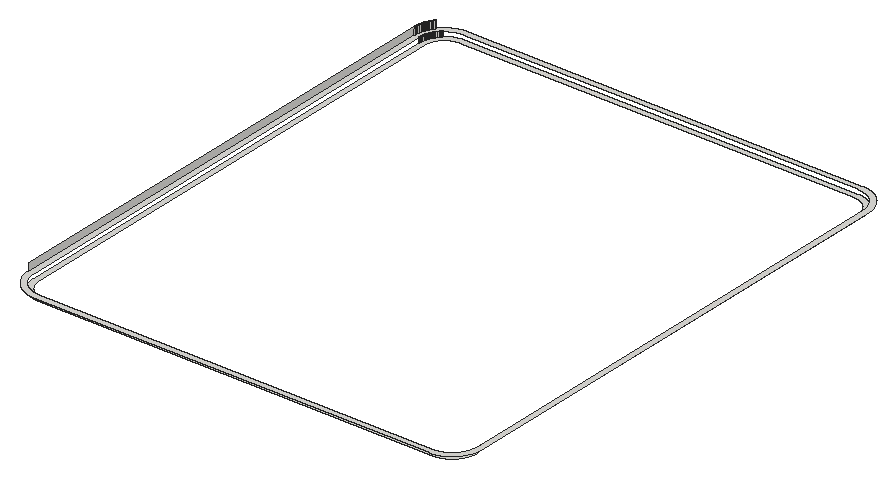
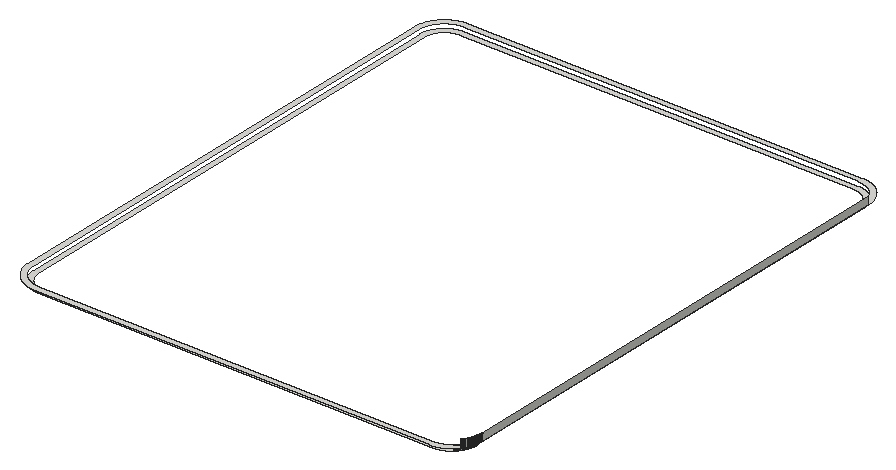
# SketchUp Ruby script. Lengths in inches.
U = 1.inch
M = Sketchup.active_model
def pt(a) = Geom::Point3d.new(a.map { |v| v * U })
def face(e, loops, mat)
  f = e.add_face(loops[0].map { |a| pt(a) })
  loops[1..].each { |l| e.add_face(l.map { |a| pt(a) }).erase! }
  f.material = f.back_material = mat if mat
  f
end
# faces: each face lists its corners as indices into pts; further lists are holes
def faces(e, pts, list, mat = nil) = list.each { |f| face(e, (f[0].is_a?(Array) ? f : [f]).map { |l| l.map { |i| pts[i] } }, mat) }
# xy, xz, yz: faces in a plane at the given z, y or x. An outline is a flat list of corners, or four numbers for a rectangle; further outlines are holes
def ring(l) = l.size == 4 ? [[l[0], l[1]], [l[2], l[1]], [l[2], l[3]], [l[0], l[3]]] : l.each_slice(2).to_a
def flat(e, list, mat, &to3) = list.each { |f| face(e, (f[0].is_a?(Array) ? f : [f]).map { |l| ring(l).map { |u, v| to3.(u, v) } }, mat) }
def xy(e, z, list, mat = nil) = flat(e, list, mat) { |x, y| [x, y, z] }
def xz(e, y, list, mat = nil) = flat(e, list, mat) { |x, z| [x, y, z] }
def yz(e, x, list, mat = nil) = flat(e, list, mat) { |y, z| [x, y, z] }
def lines(e, pts, list) = list.each { |a, b| e.add_line(pt(pts[a]), pt(pts[b])) }
# prism: a flat outline (further loops are holes) pulled along v
def prism(e, loops, v, mat = nil)
  f = face(e, loops, mat); d = Geom::Vector3d.new(v.map { |x| x * U })
  f.pushpull(f.normal.samedirection?(d) ? d.length : -d.length)
end
def box(e, o, s, mat = nil) = prism(e, [[o, [o[0] + s[0], o[1], o[2]], [o[0] + s[0], o[1] + s[1], o[2]], [o[0], o[1] + s[1], o[2]]]], [0, 0, s[2]], mat)
def at(x, y, z, deg = 0) = Geom::Transformation.translation(pt([x, y, z])) * Geom::Transformation.rotation(ORIGIN, Z_AXIS, deg.degrees)
def axes(o, x, y, z) = Geom::Transformation.new([*x, 0, *y, 0, *z, 0, *pt(o).to_a, 1])
def part(name) = M.definitions.add(name)
# library, detail: a bought-in or finely detailed component or shape, given as its bounding box
def library(name, o, s) = part(name).tap { |d| box(d.entities, o, s) }
def detail(e, o, s) = box(e.add_group.entities, o, s)
def put(e, d, t, mat = nil) = e.add_instance(d, t).tap { |i| i.material = mat if mat }
def group(e, t, mat = nil) = e.add_group.tap { |g| g.transformation = t; g.material = mat if mat }.entities
root = M.entities
M.materials.add("[Formica Graystone]").color = [224, 223, 219]
xy(root,422.82,[[[17.74,231,17.61,231.01,17.48,231.01,17.22,231.03,17.08,231.04,16.95,231.05,16.69,231.09,16.57,231.1,16.4375,231.125,16.31,231.14,16.18,231.17,16.05,231.19,15.79,231.25,15.67,231.28,15.41,231.34,15.29,231.375,15.16,231.41,15.03,231.45,14.79,231.53,14.66,231.57,14.54,231.62,14.42,231.66,14.29,231.71,14.17,231.76,14.05,231.8125,13.93,231.86,13.8125,231.92,13.69,231.97,13.58,232.03,13.34,232.15,13.23,232.21,13.11,232.28,13,232.34,12.89,232.41,12.78,232.47,12.66,232.54,12.55,232.61,12.44,232.69,12.34,232.76,12.23,232.83,12.12,232.91,12.02,232.99,11.91,233.07,11.71,233.23,11.61,233.3125,11.51,233.4,11.41,233.48,11.21,233.66,11.12,233.75,11.02,233.84,10.84,234.02,10.75,234.12,10.66,234.21,10.48,234.41,10.4,234.51,10.3125,234.61,10.23,234.71,10.07,234.91,9.99,235.02,9.91,235.12,9.83,235.23,9.76,235.34,9.69,235.44,9.61,235.55,9.54,235.66,9.47,235.78,9.41,235.89,9.34,236,9.28,236.11,9.21,236.23,9.15,236.34,9.03,236.58,8.97,236.69,8.92,236.8125,8.86,236.93,8.8125,237.05,8.76,237.17,8.71,237.29,8.66,237.42,8.62,237.54,8.57,237.66,8.53,237.79,8.45,238.03,8.41,238.16,8.375,238.29,8.34,238.41,8.28,238.67,8.25,238.79,8.19,239.05,8.17,239.18,8.14,239.31,8.125,239.4375,8.1,239.57,8.09,239.69,8.05,239.95,8.04,240.08,8.03,240.22,8.01,240.48,8.01,240.61,8,240.74,8,432.26,8.01,432.39,8.01,432.52,8.03,432.78,8.04,432.92,8.05,433.05,8.09,433.31,8.1,433.43,8.125,433.5625,8.14,433.69,8.17,433.82,8.19,433.95,8.25,434.21,8.28,434.33,8.34,434.59,8.375,434.71,8.41,434.84,8.45,434.97,8.53,435.21,8.57,435.34,8.62,435.46,8.66,435.58,8.71,435.71,8.76,435.83,8.8125,435.95,8.86,436.07,8.92,436.1875,8.97,436.31,9.03,436.42,9.15,436.66,9.21,436.77,9.28,436.89,9.34,437,9.41,437.11,9.47,437.22,9.54,437.34,9.61,437.45,9.69,437.56,9.76,437.66,9.83,437.77,9.91,437.88,9.99,437.98,10.07,438.09,10.23,438.29,10.3125,438.39,10.4,438.49,10.48,438.59,10.66,438.79,10.75,438.88,10.84,438.98,11.02,439.16,11.12,439.25,11.21,439.34,11.41,439.52,11.51,439.6,11.61,439.6875,11.71,439.77,11.91,439.93,12.02,440.01,12.12,440.09,12.23,440.17,12.34,440.24,12.44,440.31,12.55,440.39,12.66,440.46,12.78,440.53,12.89,440.59,13,440.66,13.11,440.72,13.23,440.79,13.34,440.85,13.58,440.97,13.69,441.03,13.8125,441.08,13.93,441.14,14.05,441.1875,14.17,441.24,14.29,441.29,14.42,441.34,14.54,441.38,14.66,441.43,14.79,441.47,15.03,441.55,15.16,441.59,15.29,441.625,15.41,441.66,15.67,441.72,15.79,441.75,16.05,441.81,16.18,441.83,16.31,441.86,16.4375,441.875,16.57,441.9,16.69,441.91,16.95,441.95,17.08,441.96,17.22,441.97,17.48,441.99,17.61,441.99,17.74,442,174.26,442,174.39,441.99,174.52,441.99,174.78,441.97,174.92,441.96,175.05,441.95,175.31,441.91,175.43,441.9,175.5625,441.875,175.69,441.86,175.82,441.83,175.95,441.81,176.21,441.75,176.33,441.72,176.59,441.66,176.71,441.625,176.84,441.59,176.97,441.55,177.21,441.47,177.34,441.43,177.46,441.38,177.58,441.34,177.71,441.29,177.83,441.24,177.95,441.1875,178.07,441.14,178.1875,441.08,178.31,441.03,178.42,440.97,178.66,440.85,178.77,440.79,178.89,440.72,179,440.66,179.11,440.59,179.22,440.53,179.34,440.46,179.45,440.39,179.56,440.31,179.66,440.24,179.77,440.17,179.88,440.09,179.98,440.01,180.09,439.93,180.29,439.77,180.39,439.6875,180.49,439.6,180.59,439.52,180.79,439.34,180.88,439.25,180.98,439.16,181.16,438.98,181.25,438.88,181.34,438.79,181.52,438.59,181.6,438.49,181.6875,438.39,181.77,438.29,181.93,438.09,182.01,437.98,182.09,437.88,182.17,437.77,182.24,437.66,182.31,437.56,182.39,437.45,182.46,437.34,182.53,437.22,182.59,437.11,182.66,437,182.72,436.89,182.79,436.77,182.85,436.66,182.97,436.42,183.03,436.31,183.08,436.1875,183.14,436.07,183.1875,435.95,183.24,435.83,183.29,435.71,183.34,435.58,183.38,435.46,183.43,435.34,183.47,435.21,183.55,434.97,183.59,434.84,183.625,434.71,183.66,434.59,183.72,434.33,183.75,434.21,183.81,433.95,183.83,433.82,183.86,433.69,183.875,433.5625,183.9,433.43,183.91,433.31,183.95,433.05,183.96,432.92,183.97,432.78,183.99,432.52,183.99,432.39,184,432.26,184,240.74,183.99,240.61,183.99,240.48,183.97,240.22,183.96,240.08,183.95,239.95,183.91,239.69,183.9,239.57,183.875,239.4375,183.86,239.31,183.83,239.18,183.81,239.05,183.75,238.79,183.72,238.67,183.66,238.41,183.625,238.29,183.59,238.16,183.55,238.03,183.47,237.79,183.43,237.66,183.38,237.54,183.34,237.42,183.29,237.29,183.24,237.17,183.1875,237.05,183.14,236.93,183.08,236.8125,183.03,236.69,182.97,236.58,182.85,236.34,182.79,236.23,182.72,236.11,182.66,236,182.59,235.89,182.53,235.78,182.46,235.66,182.39,235.55,182.31,235.44,182.24,235.34,182.17,235.23,182.09,235.12,182.01,235.02,181.93,234.91,181.77,234.71,181.6875,234.61,181.6,234.51,181.52,234.41,181.34,234.21,181.25,234.12,181.16,234.02,180.98,233.84,180.88,233.75,180.79,233.66,180.59,233.48,180.49,233.4,180.39,233.3125,180.29,233.23,180.09,233.07,179.98,232.99,179.88,232.91,179.77,232.83,179.66,232.76,179.56,232.69,179.45,232.61,179.34,232.54,179.22,232.47,179.11,232.41,179,232.34,178.89,232.28,178.77,232.21,178.66,232.15,178.42,232.03,178.31,231.97,178.1875,231.92,178.07,231.86,177.95,231.8125,177.83,231.76,177.71,231.71,177.58,231.66,177.46,231.62,177.34,231.57,177.21,231.53,176.97,231.45,176.84,231.41,176.71,231.375,176.59,231.34,176.33,231.28,176.21,231.25,175.95,231.19,175.82,231.17,175.69,231.14,175.5625,231.125,175.43,231.1,175.31,231.09,175.05,231.05,174.92,231.04,174.78,231.03,174.52,231.01,174.39,231.01,174.26,231],[17.79,233,174.21,233,174.3125,233.01,174.42,233.01,174.52,233.02,174.63,233.02,174.73,233.03,174.84,233.04,174.94,233.06,175.04,233.07,175.15,233.08,175.35,233.12,175.46,233.13,175.5625,233.15,175.66,233.17,175.77,233.2,175.87,233.22,175.97,233.25,176.07,233.27,176.57,233.42,176.67,233.46,176.77,233.49,176.87,233.53,176.96,233.57,177.0625,233.61,177.16,233.65,177.25,233.69,177.35,233.73,177.44,233.78,177.54,233.83,177.63,233.87,177.72,233.92,177.82,233.97,178,234.07,178.18,234.18,178.27,234.23,178.36,234.29,178.44,234.35,178.62,234.47,178.7,234.53,178.79,234.59,178.87,234.65,178.95,234.72,179.03,234.78,179.12,234.85,179.2,234.92,179.27,234.99,179.35,235.05,179.51,235.2,179.58,235.27,179.66,235.34,179.73,235.42,179.8,235.49,179.95,235.65,180.01,235.73,180.08,235.8,180.15,235.88,180.22,235.97,180.28,236.05,180.35,236.13,180.41,236.21,180.47,236.3,180.53,236.38,180.65,236.56,180.71,236.64,180.77,236.73,180.82,236.82,180.93,237,181.03,237.18,181.08,237.28,181.13,237.37,181.17,237.46,181.22,237.56,181.27,237.65,181.31,237.75,181.35,237.84,181.39,237.9375,181.43,238.04,181.47,238.13,181.51,238.23,181.54,238.33,181.58,238.43,181.73,238.93,181.75,239.03,181.78,239.13,181.8,239.23,181.83,239.34,181.85,239.4375,181.87,239.54,181.88,239.65,181.92,239.85,181.93,239.96,181.94,240.06,181.96,240.16,181.97,240.27,181.98,240.37,181.98,240.48,181.99,240.58,181.99,240.6875,182,240.79,182,432.21,181.99,432.3125,181.99,432.42,181.98,432.52,181.98,432.63,181.97,432.73,181.96,432.84,181.94,432.94,181.93,433.04,181.92,433.15,181.88,433.35,181.87,433.46,181.85,433.5625,181.83,433.66,181.8,433.77,181.78,433.87,181.75,433.97,181.73,434.07,181.58,434.57,181.54,434.67,181.51,434.77,181.47,434.87,181.43,434.96,181.39,435.0625,181.35,435.16,181.31,435.25,181.27,435.35,181.22,435.44,181.17,435.54,181.13,435.63,181.08,435.72,181.03,435.82,180.93,436,180.82,436.18,180.77,436.27,180.71,436.36,180.65,436.44,180.53,436.62,180.47,436.7,180.41,436.79,180.35,436.87,180.28,436.95,180.22,437.03,180.15,437.12,180.08,437.2,180.01,437.27,179.95,437.35,179.8,437.51,179.73,437.58,179.66,437.66,179.58,437.73,179.51,437.8,179.35,437.95,179.27,438.01,179.2,438.08,179.12,438.15,179.03,438.22,178.95,438.28,178.87,438.35,178.79,438.41,178.7,438.47,178.62,438.53,178.44,438.65,178.36,438.71,178.27,438.77,178.18,438.82,178,438.93,177.82,439.03,177.72,439.08,177.63,439.13,177.54,439.17,177.44,439.22,177.35,439.27,177.25,439.31,177.16,439.35,177.0625,439.39,176.96,439.43,176.87,439.47,176.77,439.51,176.67,439.54,176.57,439.58,176.07,439.73,175.97,439.75,175.87,439.78,175.77,439.8,175.66,439.83,175.5625,439.85,175.46,439.87,175.35,439.88,175.15,439.92,175.04,439.93,174.94,439.94,174.84,439.96,174.73,439.97,174.63,439.98,174.52,439.98,174.42,439.99,174.3125,439.99,174.21,440,17.79,440,17.6875,439.99,17.58,439.99,17.48,439.98,17.37,439.98,17.27,439.97,17.16,439.96,17.06,439.94,16.96,439.93,16.85,439.92,16.65,439.88,16.54,439.87,16.4375,439.85,16.34,439.83,16.23,439.8,16.13,439.78,16.03,439.75,15.93,439.73,15.43,439.58,15.33,439.54,15.23,439.51,15.13,439.47,15.04,439.43,14.9375,439.39,14.84,439.35,14.75,439.31,14.65,439.27,14.56,439.22,14.46,439.17,14.37,439.13,14.28,439.08,14.18,439.03,14,438.93,13.82,438.82,13.73,438.77,13.64,438.71,13.56,438.65,13.38,438.53,13.3,438.47,13.21,438.41,13.13,438.35,13.05,438.28,12.97,438.22,12.88,438.15,12.8,438.08,12.73,438.01,12.65,437.95,12.49,437.8,12.42,437.73,12.34,437.66,12.27,437.58,12.2,437.51,12.05,437.35,11.99,437.27,11.92,437.2,11.85,437.12,11.78,437.03,11.72,436.95,11.65,436.87,11.59,436.79,11.53,436.7,11.47,436.62,11.35,436.44,11.29,436.36,11.23,436.27,11.18,436.18,11.07,436,10.97,435.82,10.92,435.72,10.87,435.63,10.83,435.54,10.78,435.44,10.73,435.35,10.69,435.25,10.65,435.16,10.61,435.0625,10.57,434.96,10.53,434.87,10.49,434.77,10.46,434.67,10.42,434.57,10.27,434.07,10.25,433.97,10.22,433.87,10.2,433.77,10.17,433.66,10.15,433.5625,10.13,433.46,10.12,433.35,10.08,433.15,10.07,433.04,10.06,432.94,10.04,432.84,10.03,432.73,10.02,432.63,10.02,432.52,10.01,432.42,10.01,432.3125,10,432.21,10,240.79,10.01,240.6875,10.01,240.58,10.02,240.48,10.02,240.37,10.03,240.27,10.04,240.16,10.06,240.06,10.07,239.96,10.08,239.85,10.12,239.65,10.13,239.54,10.15,239.4375,10.17,239.34,10.2,239.23,10.22,239.13,10.25,239.03,10.27,238.93,10.42,238.43,10.46,238.33,10.49,238.23,10.53,238.13,10.57,238.04,10.61,237.9375,10.65,237.84,10.69,237.75,10.73,237.65,10.78,237.56,10.83,237.46,10.87,237.37,10.92,237.28,10.97,237.18,11.07,237,11.18,236.82,11.23,236.73,11.29,236.64,11.35,236.56,11.47,236.38,11.53,236.3,11.59,236.21,11.65,236.13,11.72,236.05,11.78,235.97,11.85,235.88,11.92,235.8,11.99,235.73,12.05,235.65,12.2,235.49,12.27,235.42,12.34,235.34,12.42,235.27,12.49,235.2,12.65,235.05,12.73,234.99,12.8,234.92,12.88,234.85,12.97,234.78,13.05,234.72,13.13,234.65,13.21,234.59,13.3,234.53,13.38,234.47,13.56,234.35,13.64,234.29,13.73,234.23,13.82,234.18,14,234.07,14.18,233.97,14.28,233.92,14.37,233.87,14.46,233.83,14.56,233.78,14.65,233.73,14.75,233.69,14.84,233.65,14.9375,233.61,15.04,233.57,15.13,233.53,15.23,233.49,15.33,233.46,15.43,233.42,15.93,233.27,16.03,233.25,16.13,233.22,16.23,233.2,16.34,233.17,16.4375,233.15,16.54,233.13,16.65,233.12,16.85,233.08,16.96,233.07,17.06,233.06,17.16,233.04,17.27,233.03,17.37,233.02,17.48,233.02,17.58,233.01,17.6875,233.01]]],"[Formica Graystone]")
xy(root,424.82,[[[17.6875,229,17.53,229.01,17.37,229.02,17.22,229.03,16.9,229.05,16.75,229.07,16.59,229.08,16.43,229.1,16.28,229.125,16.12,229.15,15.97,229.17,15.8125,229.2,15.66,229.23,15.51,229.26,15.35,229.3,15.2,229.33,15.05,229.37,14.89,229.41,14.59,229.49,14.14,229.64,13.99,229.6875,13.85,229.74,13.7,229.8,13.55,229.85,13.41,229.91,13.26,229.97,13.12,230.04,12.98,230.1,12.83,230.17,12.27,230.45,12.14,230.53,12,230.61,11.86,230.6875,11.73,230.77,11.6,230.85,11.46,230.9375,11.33,231.02,11.07,231.2,10.95,231.29,10.82,231.38,10.69,231.48,10.57,231.58,10.45,231.67,10.33,231.77,10.09,231.98,9.97,232.08,9.85,232.1875,9.74,232.3,9.625,232.4,9.51,232.51,9.4,232.625,9.3,232.74,9.1875,232.85,9.08,232.97,8.98,233.09,8.77,233.33,8.67,233.45,8.58,233.57,8.48,233.69,8.38,233.82,8.29,233.95,8.2,234.07,8.02,234.33,7.9375,234.46,7.85,234.6,7.77,234.73,7.6875,234.86,7.61,235,7.53,235.14,7.45,235.27,7.17,235.83,7.1,235.98,7.04,236.12,6.97,236.26,6.91,236.41,6.85,236.55,6.8,236.7,6.74,236.85,6.6875,236.99,6.64,237.14,6.49,237.59,6.41,237.89,6.37,238.05,6.33,238.2,6.3,238.35,6.26,238.51,6.23,238.66,6.2,238.8125,6.17,238.97,6.15,239.12,6.125,239.28,6.1,239.43,6.08,239.59,6.07,239.75,6.05,239.9,6.03,240.22,6.02,240.37,6.01,240.53,6,240.6875,6,432.3125,6.01,432.47,6.02,432.63,6.03,432.78,6.05,433.1,6.07,433.25,6.08,433.41,6.1,433.57,6.125,433.72,6.15,433.88,6.17,434.03,6.2,434.1875,6.23,434.34,6.26,434.49,6.3,434.65,6.33,434.8,6.37,434.95,6.41,435.11,6.49,435.41,6.64,435.86,6.6875,436.01,6.74,436.15,6.8,436.3,6.85,436.45,6.91,436.59,6.97,436.74,7.04,436.88,7.1,437.02,7.17,437.17,7.45,437.73,7.53,437.86,7.61,438,7.6875,438.14,7.77,438.27,7.85,438.4,7.9375,438.54,8.02,438.67,8.2,438.93,8.29,439.05,8.38,439.18,8.48,439.31,8.58,439.43,8.67,439.55,8.77,439.67,8.98,439.91,9.08,440.03,9.1875,440.15,9.3,440.26,9.4,440.375,9.51,440.49,9.625,440.6,9.74,440.7,9.85,440.8125,9.97,440.92,10.09,441.02,10.33,441.23,10.45,441.33,10.57,441.42,10.69,441.52,10.82,441.62,10.95,441.71,11.07,441.8,11.33,441.98,11.46,442.0625,11.6,442.15,11.73,442.23,11.86,442.3125,12,442.39,12.14,442.47,12.27,442.55,12.83,442.83,12.98,442.9,13.12,442.96,13.26,443.03,13.41,443.09,13.55,443.15,13.7,443.2,13.85,443.26,13.99,443.3125,14.14,443.36,14.59,443.51,14.89,443.59,15.05,443.63,15.2,443.67,15.35,443.7,15.51,443.74,15.66,443.77,15.8125,443.8,15.97,443.83,16.12,443.85,16.28,443.875,16.43,443.9,16.59,443.92,16.75,443.93,16.9,443.95,17.22,443.97,17.37,443.98,17.53,443.99,17.6875,444,174.3125,444,174.47,443.99,174.63,443.98,174.78,443.97,175.1,443.95,175.25,443.93,175.41,443.92,175.57,443.9,175.72,443.875,175.88,443.85,176.03,443.83,176.1875,443.8,176.34,443.77,176.49,443.74,176.65,443.7,176.8,443.67,176.95,443.63,177.11,443.59,177.41,443.51,177.86,443.36,178.01,443.3125,178.15,443.26,178.3,443.2,178.45,443.15,178.59,443.09,178.74,443.03,178.88,442.96,179.02,442.9,179.17,442.83,179.73,442.55,179.86,442.47,180,442.39,180.14,442.3125,180.27,442.23,180.4,442.15,180.54,442.0625,180.67,441.98,180.93,441.8,181.05,441.71,181.18,441.62,181.31,441.52,181.43,441.42,181.55,441.33,181.67,441.23,181.91,441.02,182.03,440.92,182.15,440.8125,182.26,440.7,182.375,440.6,182.49,440.49,182.6,440.375,182.7,440.26,182.8125,440.15,182.92,440.03,183.02,439.91,183.23,439.67,183.33,439.55,183.42,439.43,183.52,439.31,183.62,439.18,183.71,439.05,183.8,438.93,183.98,438.67,184.0625,438.54,184.15,438.4,184.23,438.27,184.3125,438.14,184.39,438,184.47,437.86,184.55,437.73,184.83,437.17,184.9,437.02,184.96,436.88,185.03,436.74,185.09,436.59,185.15,436.45,185.2,436.3,185.26,436.15,185.3125,436.01,185.36,435.86,185.51,435.41,185.59,435.11,185.63,434.95,185.67,434.8,185.7,434.65,185.74,434.49,185.77,434.34,185.8,434.1875,185.83,434.03,185.85,433.88,185.875,433.72,185.9,433.57,185.92,433.41,185.93,433.25,185.95,433.1,185.97,432.78,185.98,432.63,185.99,432.47,186,432.3125,186,240.6875,185.99,240.53,185.98,240.37,185.97,240.22,185.95,239.9,185.93,239.75,185.92,239.59,185.9,239.43,185.875,239.28,185.85,239.12,185.83,238.97,185.8,238.8125,185.77,238.66,185.74,238.51,185.7,238.35,185.67,238.2,185.63,238.05,185.59,237.89,185.51,237.59,185.36,237.14,185.3125,236.99,185.26,236.85,185.2,236.7,185.15,236.55,185.09,236.41,185.03,236.26,184.96,236.12,184.9,235.98,184.83,235.83,184.55,235.27,184.47,235.14,184.39,235,184.3125,234.86,184.23,234.73,184.15,234.6,184.0625,234.46,183.98,234.33,183.8,234.07,183.71,233.95,183.62,233.82,183.52,233.69,183.42,233.57,183.33,233.45,183.23,233.33,183.02,233.09,182.92,232.97,182.8125,232.85,182.7,232.74,182.6,232.625,182.49,232.51,182.375,232.4,182.26,232.3,182.15,232.1875,182.03,232.08,181.91,231.98,181.67,231.77,181.55,231.67,181.43,231.58,181.31,231.48,181.18,231.38,181.05,231.29,180.93,231.2,180.67,231.02,180.54,230.9375,180.4,230.85,180.27,230.77,180.14,230.6875,180,230.61,179.86,230.53,179.73,230.45,179.17,230.17,179.02,230.1,178.88,230.04,178.74,229.97,178.59,229.91,178.45,229.85,178.3,229.8,178.15,229.74,178.01,229.6875,177.86,229.64,177.41,229.49,177.11,229.41,176.95,229.37,176.8,229.33,176.65,229.3,176.49,229.26,176.34,229.23,176.1875,229.2,176.03,229.17,175.88,229.15,175.72,229.125,175.57,229.1,175.41,229.08,175.25,229.07,175.1,229.05,174.78,229.03,174.63,229.02,174.47,229.01,174.3125,229],[17.74,231,174.26,231,174.39,231.01,174.52,231.01,174.78,231.03,174.92,231.04,175.05,231.05,175.31,231.09,175.43,231.1,175.5625,231.125,175.69,231.14,175.82,231.17,175.95,231.19,176.21,231.25,176.33,231.28,176.59,231.34,176.71,231.375,176.84,231.41,176.97,231.45,177.21,231.53,177.34,231.57,177.46,231.62,177.58,231.66,177.71,231.71,177.83,231.76,177.95,231.8125,178.07,231.86,178.1875,231.92,178.31,231.97,178.42,232.03,178.66,232.15,178.77,232.21,178.89,232.28,179,232.34,179.11,232.41,179.22,232.47,179.34,232.54,179.45,232.61,179.56,232.69,179.66,232.76,179.77,232.83,179.88,232.91,179.98,232.99,180.09,233.07,180.29,233.23,180.39,233.3125,180.49,233.4,180.59,233.48,180.79,233.66,180.88,233.75,180.98,233.84,181.16,234.02,181.25,234.12,181.34,234.21,181.52,234.41,181.6,234.51,181.6875,234.61,181.77,234.71,181.93,234.91,182.01,235.02,182.09,235.12,182.17,235.23,182.24,235.34,182.31,235.44,182.39,235.55,182.46,235.66,182.53,235.78,182.59,235.89,182.66,236,182.72,236.11,182.79,236.23,182.85,236.34,182.97,236.58,183.03,236.69,183.08,236.8125,183.14,236.93,183.1875,237.05,183.24,237.17,183.29,237.29,183.34,237.42,183.38,237.54,183.43,237.66,183.47,237.79,183.55,238.03,183.59,238.16,183.625,238.29,183.66,238.41,183.72,238.67,183.75,238.79,183.81,239.05,183.83,239.18,183.86,239.31,183.875,239.4375,183.9,239.57,183.91,239.69,183.95,239.95,183.96,240.08,183.97,240.22,183.99,240.48,183.99,240.61,184,240.74,184,432.26,183.99,432.39,183.99,432.52,183.97,432.78,183.96,432.92,183.95,433.05,183.91,433.31,183.9,433.43,183.875,433.5625,183.86,433.69,183.83,433.82,183.81,433.95,183.75,434.21,183.72,434.33,183.66,434.59,183.625,434.71,183.59,434.84,183.55,434.97,183.47,435.21,183.43,435.34,183.38,435.46,183.34,435.58,183.29,435.71,183.24,435.83,183.1875,435.95,183.14,436.07,183.08,436.1875,183.03,436.31,182.97,436.42,182.85,436.66,182.79,436.77,182.72,436.89,182.66,437,182.59,437.11,182.53,437.22,182.46,437.34,182.39,437.45,182.31,437.56,182.24,437.66,182.17,437.77,182.09,437.88,182.01,437.98,181.93,438.09,181.77,438.29,181.6875,438.39,181.6,438.49,181.52,438.59,181.34,438.79,181.25,438.88,181.16,438.98,180.98,439.16,180.88,439.25,180.79,439.34,180.59,439.52,180.49,439.6,180.39,439.6875,180.29,439.77,180.09,439.93,179.98,440.01,179.88,440.09,179.77,440.17,179.66,440.24,179.56,440.31,179.45,440.39,179.34,440.46,179.22,440.53,179.11,440.59,179,440.66,178.89,440.72,178.77,440.79,178.66,440.85,178.42,440.97,178.31,441.03,178.1875,441.08,178.07,441.14,177.95,441.1875,177.83,441.24,177.71,441.29,177.58,441.34,177.46,441.38,177.34,441.43,177.21,441.47,176.97,441.55,176.84,441.59,176.71,441.625,176.59,441.66,176.33,441.72,176.21,441.75,175.95,441.81,175.82,441.83,175.69,441.86,175.5625,441.875,175.43,441.9,175.31,441.91,175.05,441.95,174.92,441.96,174.78,441.97,174.52,441.99,174.39,441.99,174.26,442,17.74,442,17.61,441.99,17.48,441.99,17.22,441.97,17.08,441.96,16.95,441.95,16.69,441.91,16.57,441.9,16.4375,441.875,16.31,441.86,16.18,441.83,16.05,441.81,15.79,441.75,15.67,441.72,15.41,441.66,15.29,441.625,15.16,441.59,15.03,441.55,14.79,441.47,14.66,441.43,14.54,441.38,14.42,441.34,14.29,441.29,14.17,441.24,14.05,441.1875,13.93,441.14,13.8125,441.08,13.69,441.03,13.58,440.97,13.34,440.85,13.23,440.79,13.11,440.72,13,440.66,12.89,440.59,12.78,440.53,12.66,440.46,12.55,440.39,12.44,440.31,12.34,440.24,12.23,440.17,12.12,440.09,12.02,440.01,11.91,439.93,11.71,439.77,11.61,439.6875,11.51,439.6,11.41,439.52,11.21,439.34,11.12,439.25,11.02,439.16,10.84,438.98,10.75,438.88,10.66,438.79,10.48,438.59,10.4,438.49,10.3125,438.39,10.23,438.29,10.07,438.09,9.99,437.98,9.91,437.88,9.83,437.77,9.76,437.66,9.69,437.56,9.61,437.45,9.54,437.34,9.47,437.22,9.41,437.11,9.34,437,9.28,436.89,9.21,436.77,9.15,436.66,9.03,436.42,8.97,436.31,8.92,436.1875,8.86,436.07,8.8125,435.95,8.76,435.83,8.71,435.71,8.66,435.58,8.62,435.46,8.57,435.34,8.53,435.21,8.45,434.97,8.41,434.84,8.375,434.71,8.34,434.59,8.28,434.33,8.25,434.21,8.19,433.95,8.17,433.82,8.14,433.69,8.125,433.5625,8.1,433.43,8.09,433.31,8.05,433.05,8.04,432.92,8.03,432.78,8.01,432.52,8.01,432.39,8,432.26,8,240.74,8.01,240.61,8.01,240.48,8.03,240.22,8.04,240.08,8.05,239.95,8.09,239.69,8.1,239.57,8.125,239.4375,8.14,239.31,8.17,239.18,8.19,239.05,8.25,238.79,8.28,238.67,8.34,238.41,8.375,238.29,8.41,238.16,8.45,238.03,8.53,237.79,8.57,237.66,8.62,237.54,8.66,237.42,8.71,237.29,8.76,237.17,8.8125,237.05,8.86,236.93,8.92,236.8125,8.97,236.69,9.03,236.58,9.15,236.34,9.21,236.23,9.28,236.11,9.34,236,9.41,235.89,9.47,235.78,9.54,235.66,9.61,235.55,9.69,235.44,9.76,235.34,9.83,235.23,9.91,235.12,9.99,235.02,10.07,234.91,10.23,234.71,10.3125,234.61,10.4,234.51,10.48,234.41,10.66,234.21,10.75,234.12,10.84,234.02,11.02,233.84,11.12,233.75,11.21,233.66,11.41,233.48,11.51,233.4,11.61,233.3125,11.71,233.23,11.91,233.07,12.02,232.99,12.12,232.91,12.23,232.83,12.34,232.76,12.44,232.69,12.55,232.61,12.66,232.54,12.78,232.47,12.89,232.41,13,232.34,13.11,232.28,13.23,232.21,13.34,232.15,13.58,232.03,13.69,231.97,13.8125,231.92,13.93,231.86,14.05,231.8125,14.17,231.76,14.29,231.71,14.42,231.66,14.54,231.62,14.66,231.57,14.79,231.53,15.03,231.45,15.16,231.41,15.29,231.375,15.41,231.34,15.67,231.28,15.79,231.25,16.05,231.19,16.18,231.17,16.31,231.14,16.4375,231.125,16.57,231.1,16.69,231.09,16.95,231.05,17.08,231.04,17.22,231.03,17.48,231.01,17.61,231.01]]],"[Formica Graystone]")
yz(root,6,[[241,424.82,432,427.82],[432,424.82,432.16,427.82],[432.16,424.82,432.3125,427.82]],"[Formica Graystone]")
yz(root,8,[[432,422.82,432.13,424.82],[432.13,422.82,432.26,424.82]],"[Formica Graystone]")
yz(root,8.01,[[432.39,422.82,432.52,424.82]],"[Formica Graystone]")
p = [[8,432.26,422.82],[8,432.26,424.82],[8.01,432.39,424.82],[8.01,432.39,422.82],[8.01,432.52,422.82],[8.01,432.52,424.82],
  [8.02,432.65,424.82],[8.02,432.65,422.82],[8.03,432.78,424.82],[8.03,432.78,422.82],[8.04,432.92,424.82],[8.04,432.92,422.82],
  [8.05,433.05,424.82],[8.05,433.05,422.82],[8.07,433.18,424.82],[8.07,433.18,422.82],[8.09,433.31,424.82],[8.09,433.31,422.82],
  [8.1,433.43,424.82],[8.1,433.43,422.82],[8.125,433.5625,424.82],[8.125,433.5625,422.82],[8.14,433.69,424.82],[8.14,433.69,422.82],
  [8.17,433.82,424.82],[8.17,433.82,422.82],[8.19,433.95,424.82],[8.19,433.95,422.82],[8.22,434.08,424.82],[8.22,434.08,422.82],
  [8.25,434.21,424.82],[8.25,434.21,422.82],[8.28,434.33,424.82],[8.28,434.33,422.82],[8.31,434.46,424.82],[8.31,434.46,422.82],
  [8.34,434.59,424.82],[8.34,434.59,422.82],[8.375,434.71,424.82],[8.375,434.71,422.82],[8.41,434.84,424.82],[8.41,434.84,422.82],
  [8.45,434.97,424.82],[8.45,434.97,422.82],[8.49,435.09,424.82],[8.49,435.09,422.82],[8.53,435.21,424.82],[8.53,435.21,422.82],
  [8.57,435.34,424.82],[8.57,435.34,422.82],[8.62,435.46,424.82],[8.62,435.46,422.82],[8.66,435.58,424.82],[8.66,435.58,422.82],
  [8.71,435.71,424.82],[8.71,435.71,422.82],[8.76,435.83,424.82],[8.76,435.83,422.82],[8.8125,435.95,424.82],[8.8125,435.95,422.82],
  [8.86,436.07,424.82],[8.86,436.07,422.82],[8.92,436.1875,424.82],[8.92,436.1875,422.82],[8.97,436.31,424.82],[8.97,436.31,422.82],
  [9.03,436.42,424.82],[9.03,436.42,422.82],[9.09,436.54,424.82],[9.09,436.54,422.82],[9.15,436.66,424.82],[9.15,436.66,422.82],
  [9.21,436.77,424.82],[9.21,436.77,422.82],[9.28,436.89,424.82],[9.28,436.89,422.82],[9.34,437,424.82],[9.34,437,422.82],
  [9.41,437.11,424.82],[9.41,437.11,422.82],[9.47,437.22,424.82],[9.47,437.22,422.82],[9.54,437.34,424.82],[9.54,437.34,422.82],
  [9.61,437.45,424.82],[9.61,437.45,422.82],[9.69,437.56,424.82],[9.69,437.56,422.82],[9.76,437.66,424.82],[9.76,437.66,422.82],
  [9.83,437.77,424.82],[9.83,437.77,422.82],[9.91,437.88,424.82],[9.91,437.88,422.82],[9.99,437.98,424.82],[9.99,437.98,422.82],
  [10.07,438.09,424.82],[10.07,438.09,422.82],[10.15,438.19,424.82],[10.15,438.19,422.82],[10.23,438.29,424.82],[10.23,438.29,422.82],
  [10.3125,438.39,424.82],[10.3125,438.39,422.82],[10.4,438.49,424.82],[10.4,438.49,422.82],[10.48,438.59,424.82],[10.48,438.59,422.82],
  [10.57,438.69,424.82],[10.57,438.69,422.82],[10.66,438.79,424.82],[10.66,438.79,422.82],[10.75,438.88,424.82],[10.75,438.88,422.82],
  [10.84,438.98,424.82],[10.84,438.98,422.82],[10.93,439.07,424.82],[10.93,439.07,422.82],[11.02,439.16,424.82],[11.02,439.16,422.82],
  [11.12,439.25,424.82],[11.12,439.25,422.82],[11.21,439.34,424.82],[11.21,439.34,422.82],[11.31,439.43,424.82],[11.31,439.43,422.82],
  [11.41,439.52,424.82],[11.41,439.52,422.82],[11.51,439.6,424.82],[11.51,439.6,422.82],[6.01,432.47,424.82],[6,432.3125,424.82],
  [6,432.3125,427.82],[6.01,432.47,427.82],[6.02,432.63,424.82],[6.02,432.63,427.82],[6.03,432.78,424.82],[6.03,432.78,427.82],
  [6.04,432.94,424.82],[6.04,432.94,427.82],[6.05,433.1,424.82],[6.05,433.1,427.82],[6.07,433.25,424.82],[6.07,433.25,427.82],
  [6.08,433.41,424.82],[6.08,433.41,427.82],[6.1,433.57,424.82],[6.1,433.57,427.82],[6.125,433.72,424.82],[6.125,433.72,427.82],
  [6.15,433.88,424.82],[6.15,433.88,427.82],[6.17,434.03,424.82],[6.17,434.03,427.82],[6.2,434.1875,424.82],[6.2,434.1875,427.82],
  [6.23,434.34,424.82],[6.23,434.34,427.82],[6.26,434.49,424.82],[6.26,434.49,427.82],[6.3,434.65,424.82],[6.3,434.65,427.82],
  [6.33,434.8,424.82],[6.33,434.8,427.82],[6.37,434.95,424.82],[6.37,434.95,427.82],[6.41,435.11,424.82],[6.41,435.11,427.82],
  [6.45,435.26,424.82],[6.45,435.26,427.82],[6.49,435.41,424.82],[6.49,435.41,427.82],[6.54,435.56,424.82],[6.54,435.56,427.82],
  [6.59,435.71,424.82],[6.59,435.71,427.82],[6.64,435.86,424.82],[6.64,435.86,427.82],[6.6875,436.01,424.82],[6.6875,436.01,427.82],
  [6.74,436.15,424.82],[6.74,436.15,427.82],[6.8,436.3,424.82],[6.8,436.3,427.82],[6.85,436.45,424.82],[6.85,436.45,427.82],
  [6.91,436.59,424.82],[6.91,436.59,427.82],[6.97,436.74,424.82],[6.97,436.74,427.82],[7.04,436.88,424.82],[7.04,436.88,427.82],
  [7.1,437.02,424.82],[7.1,437.02,427.82],[7.17,437.17,424.82],[7.17,437.17,427.82],[7.24,437.31,424.82],[7.24,437.31,427.82],
  [7.31,437.45,424.82],[7.31,437.45,427.82],[7.38,437.59,424.82],[7.38,437.59,427.82],[7.45,437.73,424.82],[7.45,437.73,427.82],
  [7.53,437.86,424.82],[7.53,437.86,427.82],[7.61,438,424.82],[7.61,438,427.82],[7.6875,438.14,424.82],[7.6875,438.14,427.82],
  [7.77,438.27,424.82],[7.77,438.27,427.82],[7.85,438.4,424.82],[7.85,438.4,427.82],[7.9375,438.54,424.82],[7.9375,438.54,427.82],
  [8.02,438.67,424.82],[8.02,438.67,427.82],[8.11,438.8,424.82],[8.11,438.8,427.82],[8.2,438.93,424.82],[8.2,438.93,427.82],
  [8.29,439.05,424.82],[8.29,439.05,427.82],[8.38,439.18,424.82],[8.38,439.18,427.82],[8.48,439.31,424.82],[8.48,439.31,427.82],
  [8.58,439.43,424.82],[8.58,439.43,427.82],[8.67,439.55,424.82],[8.67,439.55,427.82],[8,432,424.82],[8,432,427.82]]
faces(root,p,[[0,1,2,3],[4,5,6,7],[7,6,8,9],[9,8,10,11],[11,10,12,13],[13,12,14,15],[15,14,16,17],[17,16,18,19],
  [19,18,20,21],[21,20,22,23],[23,22,24,25],[25,24,26,27],[27,26,28,29],[29,28,30,31],[31,30,32,33],[33,32,34,35],
  [35,34,36,37],[37,36,38,39],[39,38,40,41],[41,40,42,43],[43,42,44,45],[45,44,46,47],[47,46,48,49],[49,48,50,51],
  [51,50,52,53],[53,52,54,55],[55,54,56,57],[57,56,58,59],[59,58,60,61],[61,60,62,63],[63,62,64,65],[65,64,66,67],
  [67,66,68,69],[69,68,70,71],[71,70,72,73],[73,72,74,75],[75,74,76,77],[77,76,78,79],[79,78,80,81],[81,80,82,83],
  [83,82,84,85],[85,84,86,87],[87,86,88,89],[89,88,90,91],[91,90,92,93],[93,92,94,95],[95,94,96,97],[97,96,98,99],
  [99,98,100,101],[101,100,102,103],[103,102,104,105],[105,104,106,107],[107,106,108,109],[109,108,110,111],[111,110,112,113],[113,112,114,115],
  [115,114,116,117],[117,116,118,119],[119,118,120,121],[121,120,122,123],[123,122,124,125],[125,124,126,127],[127,126,128,129],[130,131,132,133],
  [134,130,133,135],[136,134,135,137],[138,136,137,139],[140,138,139,141],[142,140,141,143],[144,142,143,145],[146,144,145,147],[148,146,147,149],
  [150,148,149,151],[152,150,151,153],[154,152,153,155],[156,154,155,157],[158,156,157,159],[160,158,159,161],[162,160,161,163],[164,162,163,165],
  [166,164,165,167],[168,166,167,169],[170,168,169,171],[172,170,171,173],[174,172,173,175],[176,174,175,177],[178,176,177,179],[180,178,179,181],
  [182,180,181,183],[184,182,183,185],[186,184,185,187],[188,186,187,189],[190,188,189,191],[192,190,191,193],[194,192,193,195],[196,194,195,197],
  [198,196,197,199],[200,198,199,201],[202,200,201,203],[204,202,203,205],[206,204,205,207],[208,206,207,209],[210,208,209,211],[212,210,211,213],
  [214,212,213,215],[216,214,215,217],[218,216,217,219],[220,218,219,221],[222,220,221,223],[224,222,223,225],[226,224,225,227],[228,226,227,229],
  [230,228,229,231]],"[Formica Graystone]")
lines(root,p,[[232,233]])
